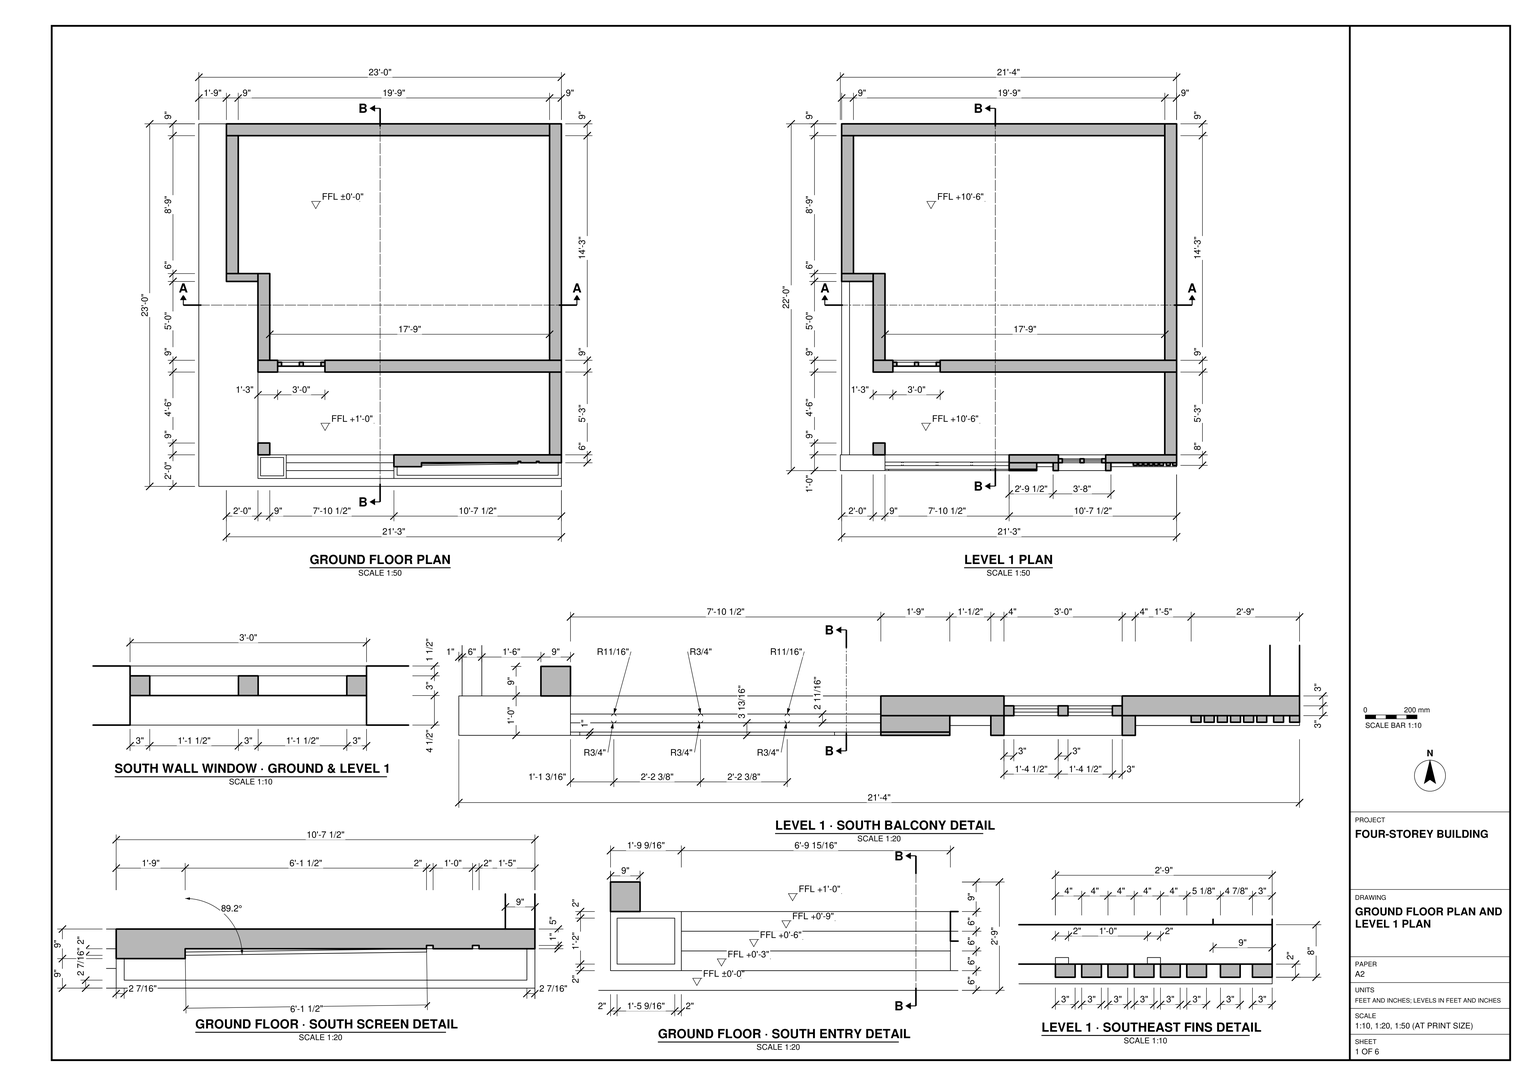
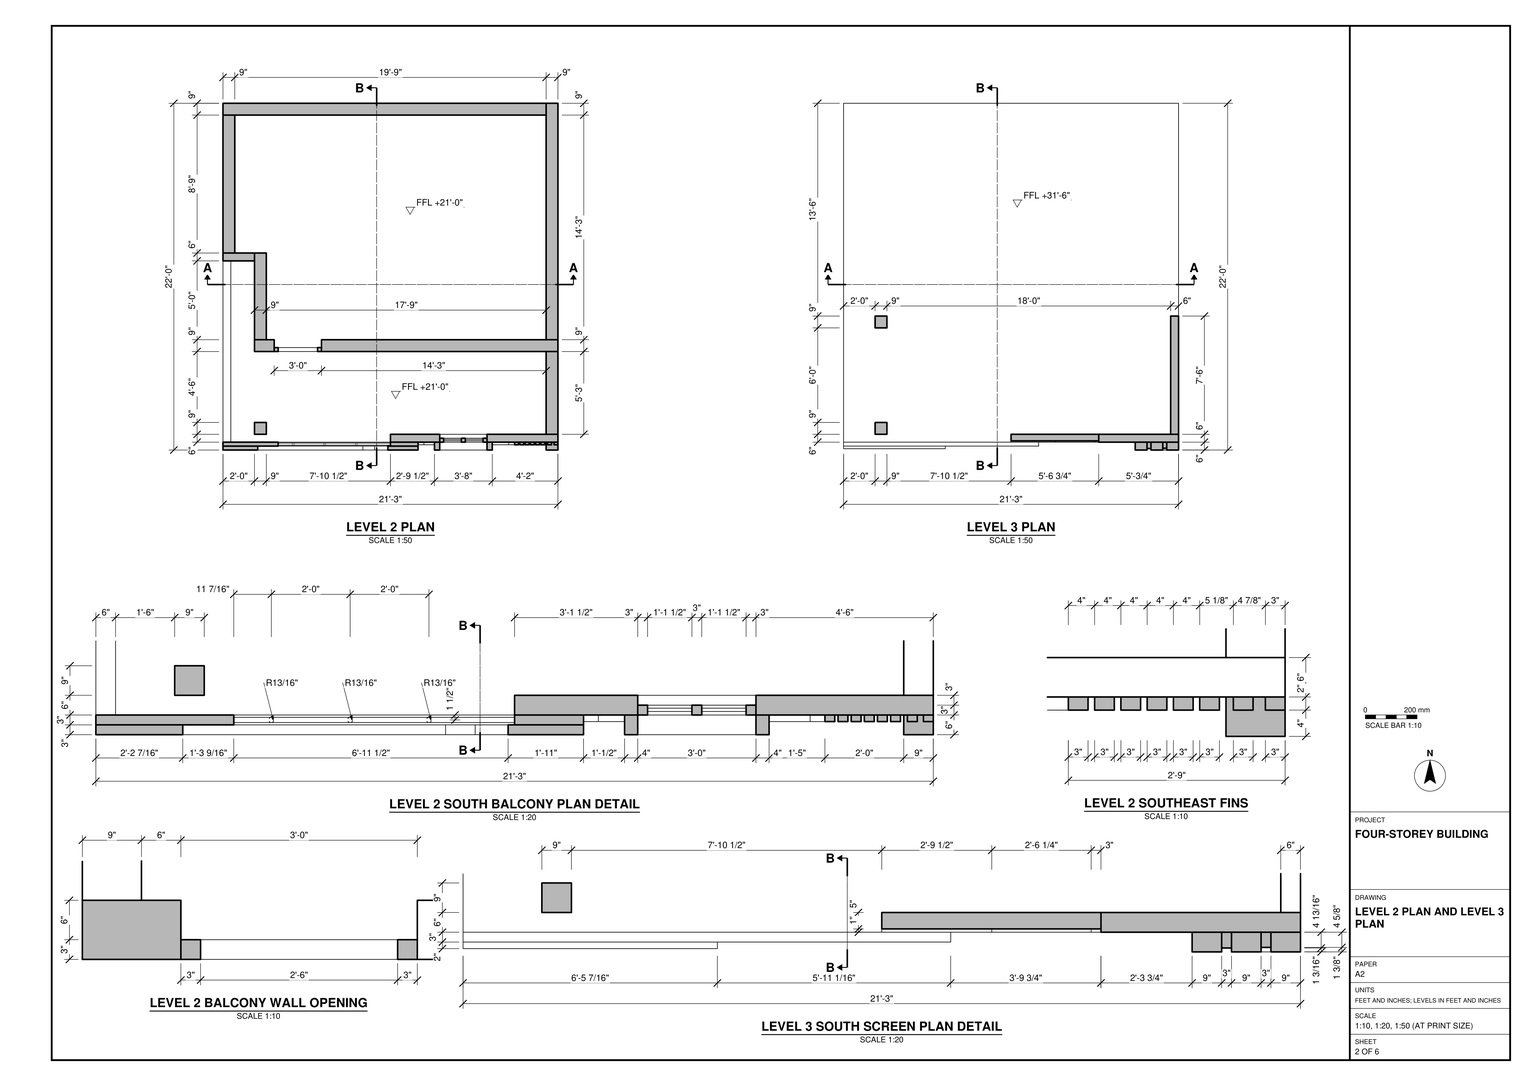
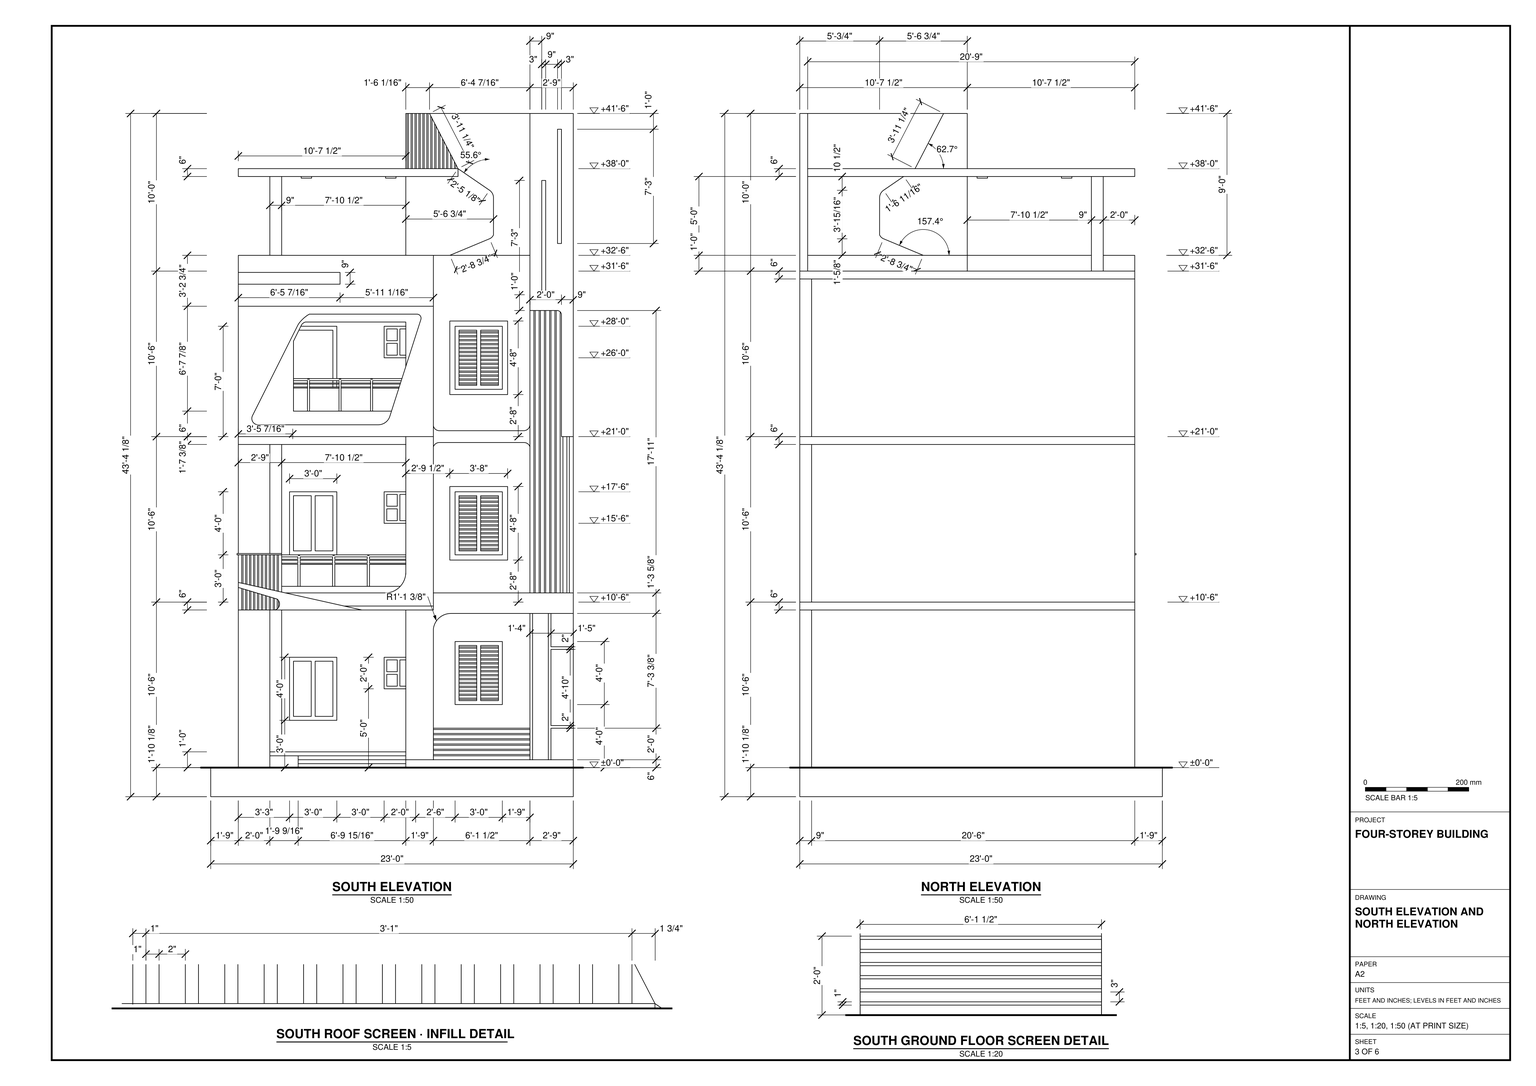
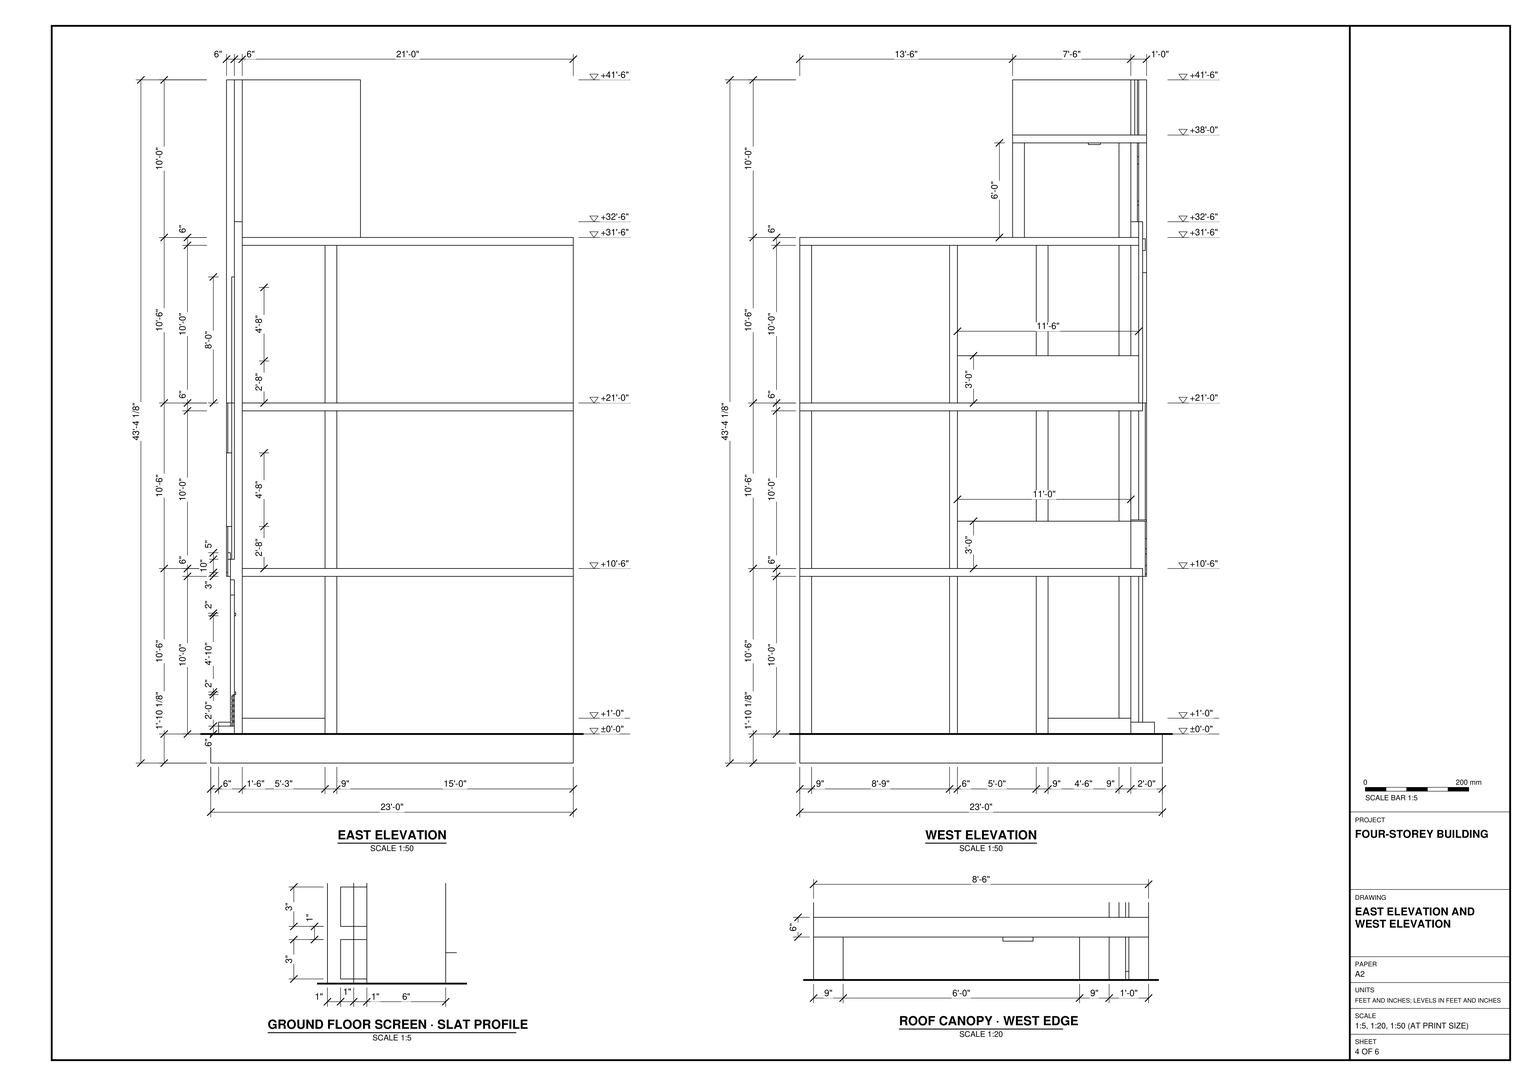
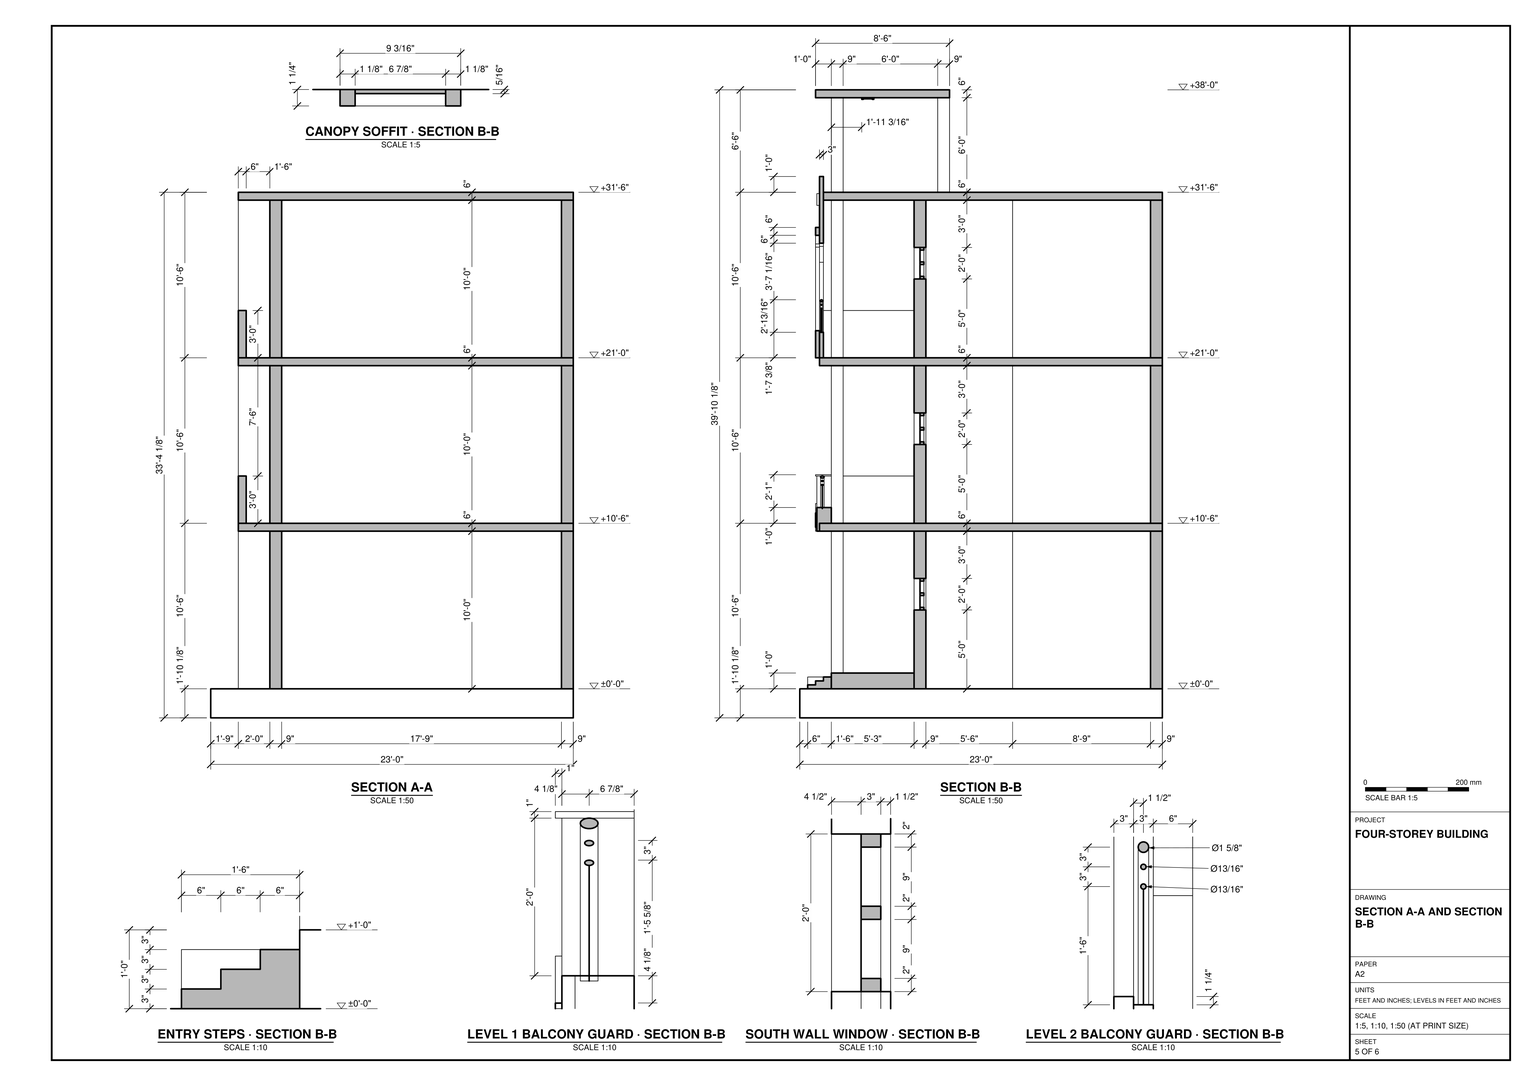
Build the four-storey building in SketchUp from task_files/diagram_01.pdf. Work in feet and inches. The overall size, from the underside of the base to the top of the roof screen, is 23'-0" wide by 23'-0" deep by 43'-4 1/8" high. Set the finished floor levels at ±0'-0", +10'-6", +21'-0" and +31'-6".

Start with the square base and use the plans to set out the slabs, walls and posts at each level. Follow the step in the west wall, using the 9" wall thickness and the 6" return where shown. On the south side, model the entry steps up to the +1'-0" landing, the recessed wall with its framed windows, and the outer screen with horizontal slats. Use the south elevation and balcony details together: the first balcony has an open railed bay, while the next has a sloping, round-cornered opening in its outer wall. Include the louvred openings and vertical fins at the east end. Keep the north wall plain below the open roof terrace, and model the terrace posts, flat canopy and raised screen.

Keep shell elements such as walls, slabs and roof, and each furniture or joinery piece shown, in separate groups or components. Use components for repeated parts. Any decor or loose items shown may be suitable library components. Save one SketchUp model as output_files/four_storey_building_with_south_balconies.skp.

# SketchUp Ruby script. Lengths in inches.
U = 1.inch
M = Sketchup.active_model
def pt(a) = Geom::Point3d.new(a.map { |v| v * U })
def face(e, loops, mat)
  f = e.add_face(loops[0].map { |a| pt(a) })
  loops[1..].each { |l| e.add_face(l.map { |a| pt(a) }).erase! }
  f.material = f.back_material = mat if mat
  f
end
# faces: each face lists its corners as indices into pts; further lists are holes
def faces(e, pts, list, mat = nil) = list.each { |f| face(e, (f[0].is_a?(Array) ? f : [f]).map { |l| l.map { |i| pts[i] } }, mat) }
# xy, xz, yz: faces in a plane at the given z, y or x. An outline is a flat list of corners, or four numbers for a rectangle; further outlines are holes
def ring(l) = l.size == 4 ? [[l[0], l[1]], [l[2], l[1]], [l[2], l[3]], [l[0], l[3]]] : l.each_slice(2).to_a
def flat(e, list, mat, &to3) = list.each { |f| face(e, (f[0].is_a?(Array) ? f : [f]).map { |l| ring(l).map { |u, v| to3.(u, v) } }, mat) }
def xy(e, z, list, mat = nil) = flat(e, list, mat) { |x, y| [x, y, z] }
def xz(e, y, list, mat = nil) = flat(e, list, mat) { |x, z| [x, y, z] }
def yz(e, x, list, mat = nil) = flat(e, list, mat) { |y, z| [x, y, z] }
def lines(e, pts, list) = list.each { |a, b| e.add_line(pt(pts[a]), pt(pts[b])) }
# prism: a flat outline (further loops are holes) pulled along v
def prism(e, loops, v, mat = nil)
  f = face(e, loops, mat); d = Geom::Vector3d.new(v.map { |x| x * U })
  f.pushpull(f.normal.samedirection?(d) ? d.length : -d.length)
end
def box(e, o, s, mat = nil) = prism(e, [[o, [o[0] + s[0], o[1], o[2]], [o[0] + s[0], o[1] + s[1], o[2]], [o[0], o[1] + s[1], o[2]]]], [0, 0, s[2]], mat)
def at(x, y, z, deg = 0) = Geom::Transformation.translation(pt([x, y, z])) * Geom::Transformation.rotation(ORIGIN, Z_AXIS, deg.degrees)
def axes(o, x, y, z) = Geom::Transformation.new([*x, 0, *y, 0, *z, 0, *pt(o).to_a, 1])
def part(name) = M.definitions.add(name)
# library, detail: a bought-in or finely detailed component or shape, given as its bounding box
def library(name, o, s) = part(name).tap { |d| box(d.entities, o, s) }
def detail(e, o, s) = box(e.add_group.entities, o, s)
def put(e, d, t, mat = nil) = e.add_instance(d, t).tap { |i| i.material = mat if mat }
def group(e, t, mat = nil) = e.add_group.tap { |g| g.transformation = t; g.material = mat if mat }.entities
root = M.entities
M.materials.add("[0047_Khaki]").color = [240, 230, 140]
M.materials.add("[0078_DarkSlateGray]").color = [47, 79, 79]
M.materials.add("[0099_LightSteelBlue]").color = [176, 196, 222]
M.materials.add("[0107_MidnightBlue]").color = [18, 18, 81]
M.materials.add("[0117_GhostWhite]").color = [248, 248, 255]
M.materials.add("[0119_RosyBrown]").color = [255, 193, 193]
M.materials.add("[0129_WhiteSmoke]").color = [245, 245, 245]
M.materials.add("[Aluminum]").color = [179, 179, 179]
M.materials.add("[Color M00]").color = [255, 255, 255]
M.materials.add("[Color M08]").color = [30, 30, 30]
M.materials.add("[Grass Dark Green]").color = [106, 157, 55]
M.materials.add("[Metal Aluminum Anodized]").color = [202, 209, 219]
M.materials.add("[Metal Rusted]").color = [184, 117, 91]
M.materials.add("[Translucent Glass Gray]").color = [0, 0, 0]
M.materials["[Translucent Glass Gray]"].alpha = 0.87
M.materials.add("[Wood Cherry Original]").color = [152, 86, 42]
M.materials.add("[Wood Veneer 02]").color = [190, 128, 91]
c1 = part("Group\#3")
box(c1.entities,[0,0,0],[24,6,120])
c2 = part("Group\#4")
box(c2.entities,[0,0,0],[9,66,120])
c3 = part("Group\#9")
prism(c3.entities,[[[231,9,0],[0,9,0],[0,9,120],[231,9,120]],[[51,9,84],[15,9,84],[15,9,36],[51,9,36]],[[111,9,84],[87,9,84],[87,9,60],[111,9,60]]],[0,-9,0])
c4 = part("Group\#6")
box(c4.entities,[0,0,0],[9,180,120])
c5 = part("Group\#7")
box(c5.entities,[0,0,0],[246,9,120])
c6 = part("Group\#2")
box(c6.entities,[0,0,0],[9,105,120])
c7 = part("Group\#17")
xz(c7.entities,0,[[3,3,16.5,45],[19.5,3,33,45]],"[Translucent Glass Gray]")
g1 = group(c7.entities,at(0,0,0),"[Wood Veneer 02]")
prism(g1,[[[0,3,0],[0,3,48],[36,3,48],[36,3,0]],[[16.5,3,3],[16.5,3,45],[3,3,45],[3,3,3]],[[33,3,45],[19.5,3,45],[19.5,3,3],[33,3,3]]],[0,-3,0])
c8 = part("Group\#11")
xz(c8.entities,0,[[2,2,10,11],[12,2,22,22],[2,13,10,22]],"[Translucent Glass Gray]")
g2 = group(c8.entities,at(0,0,0),"[Wood Veneer 02]")
prism(g2,[[[0,3,24],[24,3,24],[24,3,0],[0,3,0]],[[22,3,22],[12,3,22],[12,3,2],[22,3,2]],[[10,3,2],[10,3,11],[2,3,11],[2,3,2]],[[2,3,22],[2,3,13],[10,3,13],[10,3,22]]],[0,-3,0])
c9 = part("Group\#31")
box(c9.entities,[0,0,0],[9,9,120])
c10 = part("Group\#21")
xy(c10.entities,0,[[0,0,44,6]])
xy(c10.entities,4,[[4,0,40,6]])
xy(c10.entities,52,[[4,0,40,6]])
xy(c10.entities,56,[[0,0,44,6]])
xz(c10.entities,0,[[[0,0,44,56],[4,4,40,52]]],"[Wood Cherry Original]")
xz(c10.entities,6,[[[0,0,44,56],[4,4,40,52]]])
yz(c10.entities,0,[[0,0,6,56]])
yz(c10.entities,4,[[0,4,6,52]])
yz(c10.entities,40,[[0,4,6,52]])
yz(c10.entities,44,[[0,0,6,56]])
c11 = part("Group\#23")
prism(c11.entities,[[[0,0.98,0.37],[0,0.93,0.25],[0,0.85,0.15],[0,0.75,0.07],[0,0.63,0.02],[0,0.5,0],[0,0.37,0.02],[0,0.25,0.07],[0,0.15,0.15],[0,0.07,0.25],[0,0.02,0.37],[0,0,0.5],[0,0.02,0.63],[0,0.07,0.75],[0,0.15,0.85],[0,0.25,0.93],[0,0.37,0.98],[0,0.5,1],[0,0.63,0.98],[0,0.75,0.93],[0,0.85,0.85],[0,0.93,0.75],[0,0.98,0.63],[0,1,0.5]]],[33.3125,0,0])
c12 = part("Group\#20")
g3 = group(c12.entities,at(0,0,0),"[Color M08]")
prism(g3,[[[0,3,0],[0,3,48],[36,3,48],[36,3,0]],[[16.5,3,3],[16.5,3,45],[3,3,45],[3,3,3]],[[33,3,45],[19.5,3,45],[19.5,3,3],[33,3,3]]],[0,-3,0])
put(c12.entities,c11,at(2,1.07,6.91),"[Aluminum]")
put(c12.entities,c11,at(2,1.07,15.91),"[Aluminum]")
put(c12.entities,c11,at(2,1.07,30.91),"[Aluminum]")
put(c12.entities,c11,at(2,1.07,3.91),"[Aluminum]")
put(c12.entities,c11,at(2,1.07,39.91),"[Aluminum]")
put(c12.entities,c11,at(2,1.07,36.91),"[Aluminum]")
put(c12.entities,c11,at(2,1.07,42.91),"[Aluminum]")
put(c12.entities,c11,at(2,1.07,9.91),"[Aluminum]")
put(c12.entities,c11,at(2,1.07,24.91),"[Aluminum]")
put(c12.entities,c11,at(2,1.07,27.91),"[Aluminum]")
put(c12.entities,c11,at(2,1.07,12.91),"[Aluminum]")
put(c12.entities,c11,at(2,1.07,33.91),"[Aluminum]")
put(c12.entities,c11,at(2,1.07,18.91),"[Aluminum]")
put(c12.entities,c11,at(2,1.07,21.91),"[Aluminum]")
c13 = part("Group\#35")
box(c13.entities,[0,0,0],[1,2,42])
c14 = library("Group\#39",[192.125,0,0],[88.3125,1.6,24.79])
c15 = part("Group\#47")
box(c15.entities,[0,0,0],[3,2,215])
c16 = part("Group\#55")
xy(c16.entities,0,[[[0,0,7.9375,9.1875],[1.15,1.15,6.79,8.04]]],"[Metal Rusted]")
xy(c16.entities,0.9375,[[1.15,1.15,6.79,8.04]],"[Metal Aluminum Anodized]")
xy(c16.entities,1.25,[[[0,0,7.9375,9.1875],[1.15,1.15,6.79,8.04]]])
xz(c16.entities,0,[[0,0,7.9375,1.25]],"[Metal Rusted]")
xz(c16.entities,1.15,[[1.15,0.9375,6.79,1.25]])
xz(c16.entities,1.15,[[1.15,0,6.79,0.9375]],"[Metal Rusted]")
xz(c16.entities,8.04,[[1.15,0.9375,6.79,1.25]])
xz(c16.entities,8.04,[[1.15,0,6.79,0.9375]],"[Metal Rusted]")
xz(c16.entities,9.1875,[[0,0,7.9375,1.25]],"[Metal Rusted]")
yz(c16.entities,0,[[0,0,9.1875,1.25]])
yz(c16.entities,1.15,[[1.15,0.9375,8.04,1.25]])
yz(c16.entities,1.15,[[1.15,0,8.04,0.9375]],"[Metal Rusted]")
yz(c16.entities,6.79,[[1.15,0.9375,8.04,1.25]])
yz(c16.entities,6.79,[[1.15,0,8.04,0.9375]],"[Metal Rusted]")
yz(c16.entities,7.9375,[[0,0,9.1875,1.25]],"[Metal Rusted]")
xy(root,24.125,[[150.9375,8.4375,273.5625,8.4375,273.5625,18,148.5,18,148.5,15,150.9375,15]],"[Grass Dark Green]")
xy(root,28.125,[[148.5,6,276,6,276,18,273.5625,18,273.5625,8.4375,150.9375,8.4375,150.9375,15,148.5,15]])
xz(root,6,[[148.5,22.125,276,28.125]])
xz(root,8.4375,[[150.9375,24.125,273.5625,28.125]])
xz(root,15,[[148.5,24.125,150.9375,28.125]])
xz(root,18,[[148.5,22.125,273.5625,24.125],[273.5625,22.125,276,28.125]])
yz(root,148.5,[[6,22.125,15,28.125],[15,22.125,18,24.125]])
yz(root,150.9375,[[8.4375,24.125,15,28.125]])
yz(root,273.5625,[[8.4375,24.125,15.5625,28.125],[15.5625,24.125,18,28.125]])
yz(root,276,[[6,22.125,18,28.125]])
# 3 loose lines left out
g4 = group(root,at(36,96,0))
box(g4,[-36,-96,0],[276,276,22.125])
put(root,c1,at(21,156,22.125),"[0117_GhostWhite]")
put(root,c2,at(45,96,22.125),"[0117_GhostWhite]")
put(root,c3,at(45,87,22.125),"[0117_GhostWhite]")
put(root,c4,at(267,96,22.125),"[0117_GhostWhite]")
put(root,c5,at(21,267,22.125),"[0117_GhostWhite]")
put(root,c6,at(21,162,22.125),"[0117_GhostWhite]")
put(root,c7,at(60,91.5,58.125))
put(root,c8,at(132,91.5,82.125))
g5 = group(root,at(21,24,142.125),"[0117_GhostWhite]")
prism(g5,[[[0,-9,0],[0,252,0],[255,252,0],[255,0,0],[127.5,0,0],[127.5,-9,0]]],[0,0,6])
put(root,c6,at(21,162,148.125),"[0117_GhostWhite]")
put(root,c2,at(45,96,148.125),"[0117_GhostWhite]")
put(root,c8,at(132,91.5,208.125))
put(root,c9,at(45,24,148.125),"[0117_GhostWhite]")
put(root,c1,at(21,156,148.125),"[0117_GhostWhite]")
put(root,c5,at(21,267,148.125),"[0117_GhostWhite]")
g6 = group(root,at(21,24,268.125),"[0117_GhostWhite]")
prism(g6,[[[0,-9,0],[0,252,0],[255,252,0],[255,0,0],[127.5,0,0],[127.5,-9,0]]],[0,0,6])
put(root,c7,at(60,91.5,184.125))
put(root,c4,at(267,96,148.125),"[0117_GhostWhite]")
g7 = group(root,at(45,6,22.125),"[0117_GhostWhite]")
xy(g7,0,[[21.5625,0,103.5,18],[0,18,231,81]])
xy(g7,3,[[21.5625,0,103.5,6]])
xy(g7,6,[[21.5625,6,103.5,12]])
xy(g7,9,[[21.5625,12,103.5,18]])
xy(g7,12,[[0,18,231,81]])
xz(g7,0,[[21.5625,0,103.5,3]])
xz(g7,6,[[21.5625,3,103.5,6]])
xz(g7,12,[[21.5625,6,103.5,9]])
xz(g7,18,[[0,0,21.5625,0,21.5625,9,231,9,231,12,0,12],[21.5625,0,103.5,9],[103.5,0,231,9]])
xz(g7,81,[[0,0,231,12]])
yz(g7,0,[[18,0,81,12]])
yz(g7,21.5625,[[0,0,0,3,6,3,6,6,12,6,12,9,18,9,18,0]])
yz(g7,103.5,[[0,0,18,0,18,9,12,9,12,6,6,6,6,3,0,3]])
yz(g7,231,[[18,0,81,12]])
g8 = group(root,at(45,24,34.125),"[0117_GhostWhite]")
box(g8,[0,0,0],[9,9,108])
put(root,c6,at(21,162,274.125),"[0117_GhostWhite]")
put(root,c1,at(21,156,274.125),"[0117_GhostWhite]")
put(root,c5,at(21,267,274.125),"[0117_GhostWhite]")
g9 = group(root,at(21,24,394.125),"[0117_GhostWhite]")
prism(g9,[[[0,-6,0],[0,252,0],[255,252,0],[255,0,0],[127.5,0,0],[127.5,-6,0]]],[0,0,6])
put(root,c4,at(267,96,274.125),"[0117_GhostWhite]")
put(root,c2,at(45,96,274.125),"[0117_GhostWhite]")
g10 = group(root,at(45,87,274.125),"[0117_GhostWhite]")
g11 = group(g10,at(15,0,0),"[Wood Veneer 02]")
prism(g11,[[[0,0,0],[36,0,0],[36,0,84],[0,0,84]],[[33,0,81],[33,0,3],[3,0,3],[3,0,81]]],[0,3,0])
g12 = group(g10,at(0,0,0))
g13 = group(g12,at(0,0,0))
prism(g13,[[[51,0,84],[51,0,0],[231,0,0],[231,0,120],[0,0,120],[0,0,0],[15,0,0],[15,0,84]],[[87,0,84],[111,0,84],[111,0,60],[87,0,60]]],[0,9,0])
put(g12,c8,at(87,4.5,60))
put(root,c10,at(182,12,180.125))
put(root,c3,at(45,87,148.125),"[0117_GhostWhite]")
put(root,c12,at(186,18,184.125))
put(root,c12,at(186,18,70.125))
put(root,c12,at(186,18,310.125))
put(root,c10,at(182,12,306.125))
g14 = group(root,at(45,24,400.125),"[0117_GhostWhite]")
box(g14,[0,0,0],[9,9,72])
g15 = group(root,at(45,105,400.125),"[0117_GhostWhite]")
box(g15,[0,0,0],[9,9,72])
g16 = group(root,at(270,24,400.125),"[0117_GhostWhite]")
box(g16,[0,0,0],[6,90,120])
g17 = group(root,at(21,15,274.125),"[0119_RosyBrown]")
xy(g17,-119,[[127.5,-2,148.5,3]])
xy(g17,0,[[127.5,-2,148.5,0],[0,0,127.5,3]])
xy(g17,19.38,[[42,0,127.5,3]])
xy(g17,87.23,[[51,0,127.5,3]])
xy(g17,138,[[0,0,148.5,3]])
xz(g17,-2,[[127.5,-119,148.5,0]])
xz(g17,0,[[[0,0,148.5,138],[42,19.38,42,72.69,48,84.81,48.15,85.08,48.31,85.34,48.5,85.59,48.71,85.83,48.94,86.05,49.19,86.27,49.46,86.47,49.74,86.65,50.04,86.82,50.35,86.98,50.67,87.11,51,87.23,127.5,87.23,127.5,19.38]]])
xz(g17,3,[[[127.5,-119,127.5,0,0,0,0,138,148.5,138,148.5,-119],[42,19.38,127.5,19.38,127.5,87.23,51,87.23,50.67,87.11,50.35,86.98,50.04,86.82,49.74,86.65,49.46,86.47,49.19,86.27,48.94,86.05,48.71,85.83,48.5,85.59,48.31,85.34,48.15,85.08,48,84.81,42,72.69]]])
yz(g17,0,[[0,0,3,138]])
yz(g17,42,[[0,19.38,3,72.69]])
yz(g17,127.5,[[-2,-119,3,0],[0,19.38,3,87.23]])
yz(g17,148.5,[[-2,-119,3,-119,3,138,0,138,0,0,-2,0]])
p = [[42,3,72.69],[48,3,84.81],[48,0,84.81],[42,0,72.69],[48.15,3,85.08],[48.15,0,85.08],
  [48.31,3,85.34],[48.31,0,85.34],[48.5,3,85.59],[48.5,0,85.59],[48.71,3,85.83],[48.71,0,85.83],
  [48.94,3,86.05],[48.94,0,86.05],[49.19,3,86.27],[49.19,0,86.27],[49.46,3,86.47],[49.46,0,86.47],
  [49.74,3,86.65],[49.74,0,86.65],[50.04,3,86.82],[50.04,0,86.82],[50.35,3,86.98],[50.35,0,86.98],
  [50.67,3,87.11],[50.67,0,87.11],[51,3,87.23],[51,0,87.23]]
faces(g17,p,[[0,1,2,3],[1,4,5,2],[4,6,7,5],[6,8,9,7],[8,10,11,9],[10,12,13,11],[12,14,15,13],[14,16,17,15],
  [16,18,19,17],[18,20,21,19],[20,22,23,21],[22,24,25,23],[24,26,27,25]])
g18 = group(root,at(21,12,274.125),"[Wood Cherry Original]")
prism(g18,[[[148.5,3,99.23],[148.5,3,0],[0,3,0],[0,3,99.23]],[[47.04,3,87.33],[46.51,3,86.68],[46.08,3,86.1],[45.68,3,85.5],[45.32,3,84.875],[45,3,84.23],[10.78,3,15.95],[10.48,3,15.21],[10.31,3,14.43],[10.27,3,13.63],[10.37,3,12.84],[10.59,3,12.07],[10.9375,3,11.35],[11.4,3,10.7],[11.97,3,10.14],[12.62,3,9.67],[13.34,3,9.32],[14.1,3,9.1],[14.9,3,9],[106.5,3,9],[107.52,3,9.06],[108.52,3,9.22],[109.5,3,9.5],[110.45,3,9.88],[111.35,3,10.36],[112.1875,3,10.94],[112.96,3,11.61],[113.65,3,12.35],[114.26,3,13.17],[114.77,3,14.05],[115.1875,3,14.98],[115.5,3,15.95],[136.24,3,80.65],[137.38,3,84.23],[138.97,3,89.17],[139.08,3,89.625],[139.12,3,90.09],[139.08,3,90.56],[138.98,3,91.02],[138.82,3,91.46],[138.58,3,91.86],[138.29,3,92.23],[137.95,3,92.55],[137.57,3,92.82],[137.15,3,93.02],[136.7,3,93.16],[136.24,3,93.23],[54,3,93.23],[53.29,3,92.79],[52.59,3,92.34],[51.91,3,91.86],[51.24,3,91.36],[50.59,3,90.84],[49.95,3,90.3],[49.33,3,89.74],[48.73,3,89.17],[48.15,3,88.57],[47.58,3,87.96]]],[0,-3,0])
g19 = group(root,at(21,12,472.125))
xy(g19,0,[[0,0,0,102,249,102,249,12,167.25,12,167.25,0]])
xy(g19,6,[[0,0,167.25,0,167.25,12,249,12,249,102,0,102]])
xz(g19,0,[[0,0,167.25,6]],"[Wood Cherry Original]")
xz(g19,12,[[167.25,0,249,6]])
xz(g19,102,[[0,0,249,6]])
yz(g19,0,[[0,0,102,6]])
yz(g19,167.25,[[0,0,12,6]])
yz(g19,249,[[12,0,71.3125,6],[71.3125,0,102,6]])
g20 = group(root,at(21,13,390.13),"[0107_MidnightBlue]")
box(g20,[0,0,0],[77.4375,2,9])
g21 = group(root,at(148.5,24,412.125),"[0047_Khaki]")
xy(g21,0,[[33.5,-6,127.5,0],[0,-5,33.5,0]],"[0119_RosyBrown]")
xy(g21,60,[[0,-5,39.75,-3]],"[0119_RosyBrown]")
xy(g21,108,[[18.05,-6,127.5,0],[0,-3,18.05,0]],"[0119_RosyBrown]")
xz(g21,-6,[[33.5,0,63.75,12.62,64.08,12.77,64.4,12.9375,64.71,13.13,65,13.34,65.28,13.57,65.55,13.82,65.79,14.09,66.02,14.37,66.24,14.66,66.43,14.97,66.6,15.29,66.75,15.62,66.75,43.8,66.73,44.37,66.67,44.92,66.56,45.47,66.4,46.01,66.2,46.54,65.96,47.05,65.68,47.53,65.36,47.99,65.01,48.43,64.62,48.83,64.2,49.2,63.75,49.54,39.75,66,18.05,108,127.5,108,127.5,0]],"[0119_RosyBrown]")
xz(g21,-3,[[0,60,39.75,60,39.75,66,18.05,108,0,108]],"[0119_RosyBrown]")
xz(g21,0,[[0,0,0,108,18.05,108,39.75,66,63.75,49.54,64.2,49.2,64.62,48.83,65.01,48.43,65.36,47.99,65.68,47.53,65.96,47.05,66.2,46.54,66.4,46.01,66.56,45.47,66.67,44.92,66.73,44.37,66.75,43.8,66.75,15.62,66.6,15.29,66.43,14.97,66.24,14.66,66.02,14.37,65.79,14.09,65.55,13.82,65.28,13.57,65,13.34,64.71,13.13,64.4,12.9375,64.08,12.77,63.75,12.62,33.5,0],[33.5,0,63.75,12.62,64.08,12.77,64.4,12.9375,64.71,13.13,65,13.34,65.28,13.57,65.55,13.82,65.79,14.09,66.02,14.37,66.24,14.66,66.43,14.97,66.6,15.29,66.75,15.62,66.75,43.8,66.73,44.37,66.67,44.92,66.56,45.47,66.4,46.01,66.2,46.54,65.96,47.05,65.68,47.53,65.36,47.99,65.01,48.43,64.62,48.83,64.2,49.2,63.75,49.54,39.75,66,18.05,108,127.5,108,127.5,0]],"[0119_RosyBrown]")
yz(g21,0,[[-5,0,-5,60,-3,60,-3,108,0,108,0,0]],"[0119_RosyBrown]")
yz(g21,39.75,[[-5,60,-3,60.0625],[-5,60.0625,-3,66]],"[0119_RosyBrown]")
yz(g21,66.75,[[-6,15.62,-5,43.8],[-5,15.62,0,43.8]],"[0119_RosyBrown]")
yz(g21,127.5,[[-6,0,0,108]],"[0119_RosyBrown]")
p = [[33.5,-6,0],[63.75,-6,12.62],[63.75,-5,12.62],[33.5,-5,0],[63.75,0,12.62],[33.5,0,0],
  [64.08,-6,12.77],[64.08,-5,12.77],[64.08,0,12.77],[64.4,-6,12.9375],[64.4,-5,12.9375],[64.4,0,12.9375],
  [64.71,-6,13.13],[64.71,-5,13.13],[64.71,0,13.13],[65,-6,13.34],[65,-5,13.34],[65,0,13.34],
  [65.28,-6,13.57],[65.28,-5,13.57],[65.28,0,13.57],[65.55,-6,13.82],[65.55,-5,13.82],[65.55,0,13.82],
  [65.79,-6,14.09],[65.79,-5,14.09],[65.79,0,14.09],[66.02,-6,14.37],[66.02,-5,14.37],[66.02,0,14.37],
  [66.24,-6,14.66],[66.24,-5,14.66],[66.24,0,14.66],[66.43,-6,14.97],[66.43,-5,14.97],[66.43,0,14.97],
  [66.6,-6,15.29],[66.6,-5,15.29],[66.6,0,15.29],[66.75,-6,15.62],[66.75,-5,15.62],[66.75,0,15.62],
  [66.73,-6,44.37],[66.73,-5,44.37],[66.75,-5,43.8],[66.75,-6,43.8],[66.73,0,44.37],[66.75,0,43.8],
  [66.67,-6,44.92],[66.67,-5,44.92],[66.67,0,44.92],[66.56,-6,45.47],[66.56,-5,45.47],[66.56,0,45.47],
  [66.4,-6,46.01],[66.4,-5,46.01],[66.4,0,46.01],[66.2,-6,46.54],[66.2,-5,46.54],[66.2,0,46.54],
  [65.96,-6,47.05],[65.96,-5,47.05],[65.96,0,47.05],[65.68,-6,47.53],[65.68,-5,47.53],[65.68,0,47.53],
  [65.36,-6,47.99],[65.36,-5,47.99],[65.36,0,47.99],[65.01,-6,48.43],[65.01,-5,48.43],[65.01,0,48.43],
  [64.62,-6,48.83],[64.62,-5,48.83],[64.62,0,48.83],[64.2,-6,49.2],[64.2,-5,49.2],[64.2,0,49.2],
  [63.75,-6,49.54],[63.75,-5,49.54],[63.75,0,49.54],[39.75,-6,66],[39.75,-5,66],[39.75,0,66],
  [39.75,-3,66],[18.05,-6,108],[18.05,-3,108],[18.05,0,108]]
faces(g21,p,[[0,1,2,3],[4,5,3,2],[1,6,7,2],[8,4,2,7],[6,9,10,7],[11,8,7,10],[9,12,13,10],[14,11,10,13],
  [15,16,13,12],[17,14,13,16],[18,19,16,15],[20,17,16,19],[21,22,19,18],[23,20,19,22],[24,25,22,21],[26,23,22,25],
  [27,28,25,24],[29,26,25,28],[30,31,28,27],[32,29,28,31],[33,34,31,30],[35,32,31,34],[36,37,34,33],[38,35,34,37],
  [39,40,37,36],[41,38,37,40],[42,43,44,45],[46,47,44,43],[48,49,43,42],[50,46,43,49],[51,52,49,48],[53,50,49,52],
  [54,55,52,51],[56,53,52,55],[57,58,55,54],[59,56,55,58],[60,61,58,57],[62,59,58,61],[63,64,61,60],[65,62,61,64],
  [66,67,64,63],[68,65,64,67],[69,70,67,66],[71,68,67,70],[72,73,70,69],[74,71,70,73],[75,76,73,72],[77,74,73,76],
  [78,79,76,75],[80,77,76,79],[81,82,79,78],[83,80,79,82,84],[85,86,84,82,81],[87,83,84,86]],"[0119_RosyBrown]")
g22 = group(g21,at(0,-5,0))
xz(g22,0,[[0,0,33.5,0,63.75,12.62,64.08,12.77,64.4,12.9375,64.71,13.13,65,13.34,65.28,13.57,65.55,13.82,65.79,14.09,66.02,14.37,66.24,14.66,66.43,14.97,66.6,15.29,66.75,15.62,66.75,43.8,66.73,44.37,66.67,44.92,66.56,45.47,66.4,46.01,66.2,46.54,65.96,47.05,65.68,47.53,65.36,47.99,65.01,48.43,64.62,48.83,64.2,49.2,63.75,49.54,39.75,66,39.75,60,0,60]],"[Color M00]")
g23 = group(root,at(149.5,19,478.125),"[0119_RosyBrown]")
put(g23,c13,at(6,0,0))
put(g23,c13,at(12,0,0))
put(g23,c13,at(0,0,0))
put(g23,c13,at(30,0,0))
put(g23,c13,at(9,0,0))
put(g23,c13,at(33,0,0))
put(g23,c13,at(3,0,0))
put(g23,c13,at(27,0,0))
put(g23,c13,at(15,0,0))
put(g23,c13,at(18,0,0))
put(g23,c13,at(21,0,0))
put(g23,c13,at(36,0,0))
put(g23,c13,at(24,0,0))
put(root,c14,at(-129.6875,15.7,293.51))
g24 = group(root,at(21,18,274.125),"[0117_GhostWhite]")
box(g24,[0,0,0],[6,138,36])
g25 = group(root,at(21,24,148.125),"[0117_GhostWhite]")
box(g25,[0,0,0],[6,132,36])
put(root,c9,at(45,24,274.125))
g26 = group(root,at(21,15,148.125),"[0119_RosyBrown]")
xy(g26,-6,[[0,-2,0,0,33,0,33,-2,30.56,-2,30.56,-1,29.56,-1,29.56,-2,27.56,-2,27.56,-1,26.56,-1,26.56,-2,24.56,-2,24.56,-1,23.56,-1,23.56,-2,21.56,-2,21.56,-1,20.56,-1,20.56,-2,18.56,-2,18.56,-1,17.56,-1,17.56,-2,15.56,-2,15.56,-1,14.56,-1,14.56,-2,12.56,-2,12.56,-1,11.56,-1,11.56,-2,9.56,-2,9.56,-1,8.56,-1,8.56,-2,6.56,-2,6.56,-1,5.56,-1,5.56,-2,3.56,-2,3.56,-1,2.56,-1,2.56,-2],[33,-2,148.5,0]],"[0047_Khaki]")
xy(g26,0,[[0,0,127.5,9]],"[0047_Khaki]")
xy(g26,12,[[33,-2,148.5,-2,148.5,0,127.5,0,127.5,9,33,9]])
xy(g26,36,[[0,-2,2.56,-2,2.56,-1,3.56,-1,3.56,-2,5.56,-2,5.56,-1,6.56,-1,6.56,-2,8.56,-2,8.56,-1,9.56,-1,9.56,-2,11.56,-2,11.56,-1,12.56,-1,12.56,-2,14.56,-2,14.56,-1,15.56,-1,15.56,-2,17.56,-2,17.56,-1,18.56,-1,18.56,-2,20.56,-2,20.56,-1,21.56,-1,21.56,-2,23.56,-2,23.56,-1,24.56,-1,24.56,-2,26.56,-2,26.56,-1,27.56,-1,27.56,-2,29.56,-2,29.56,-1,30.56,-1,30.56,-2,33,-2,33,9,0,9]],"[0047_Khaki]")
xz(g26,-2,[[33,-6,148.5,12]])
xz(g26,-2,[[0,-6,2.56,36],[3.56,-6,5.56,36],[6.56,-6,8.56,36],[9.56,-6,11.56,36],[12.56,-6,14.56,36],
  [15.56,-6,17.56,36],[18.56,-6,20.56,36],[21.56,-6,23.56,36],[24.56,-6,26.56,36],[27.56,-6,29.56,36],
  [30.56,-6,33,36]],"[0047_Khaki]")
xz(g26,-1,[[2.56,-6,3.56,36],[5.56,-6,6.56,36],[8.56,-6,9.56,36],[11.56,-6,12.56,36],[14.56,-6,15.56,36],
  [17.56,-6,18.56,36],[20.56,-6,21.56,36],[23.56,-6,24.56,36],[26.56,-6,27.56,36],[29.56,-6,30.56,36]],"[0047_Khaki]")
xz(g26,0,[[0,-6,33,0],[33,-6,148.5,0],[127.5,0,148.5,12]],"[0047_Khaki]")
xz(g26,9,[[0,0,0,36,33,36,33,12,127.5,12,127.5,0]],"[0047_Khaki]")
yz(g26,0,[[-2,-6,-2,36,9,36,9,0,0,0,0,-6]],"[0047_Khaki]")
yz(g26,2.56,[[-2,-6,-1,36]],"[0047_Khaki]")
yz(g26,3.56,[[-2,-6,-1,36]],"[0047_Khaki]")
yz(g26,5.56,[[-2,-6,-1,36]],"[0047_Khaki]")
yz(g26,6.56,[[-2,-6,-1,36]],"[0047_Khaki]")
yz(g26,8.56,[[-2,-6,-1,36]],"[0047_Khaki]")
yz(g26,9.56,[[-2,-6,-1,36]],"[0047_Khaki]")
yz(g26,11.56,[[-2,-6,-1,36]],"[0047_Khaki]")
yz(g26,12.56,[[-2,-6,-1,36]],"[0047_Khaki]")
yz(g26,14.56,[[-2,-6,-1,36]],"[0047_Khaki]")
yz(g26,15.56,[[-2,-6,-1,36]],"[0047_Khaki]")
yz(g26,17.56,[[-2,-6,-1,36]],"[0047_Khaki]")
yz(g26,18.56,[[-2,-6,-1,36]],"[0047_Khaki]")
yz(g26,20.56,[[-2,-6,-1,36]],"[0047_Khaki]")
yz(g26,21.56,[[-2,-6,-1,36]],"[0047_Khaki]")
yz(g26,23.56,[[-2,-6,-1,36]],"[0047_Khaki]")
yz(g26,24.56,[[-2,-6,-1,36]],"[0047_Khaki]")
yz(g26,26.56,[[-2,-6,-1,36]],"[0047_Khaki]")
yz(g26,27.56,[[-2,-6,-1,36]],"[0047_Khaki]")
yz(g26,29.56,[[-2,-6,-1,36]],"[0047_Khaki]")
yz(g26,30.56,[[-2,-6,-1,36]],"[0047_Khaki]")
yz(g26,33,[[-2,12,9,36]])
yz(g26,33,[[-2,-6,0,12]],"[0047_Khaki]")
yz(g26,127.5,[[0,0,9,12]],"[0047_Khaki]")
yz(g26,148.5,[[-2,-6,0,12]])
g27 = group(root,at(21,12,142.125),"[0099_LightSteelBlue]")
prism(g27,[[[29.56,0,0],[33,0,0],[94.07,0,0],[0,0,21],[0,0,17.17],[29.56,0,8.31],[30.01,0,7.91],[30.4,0,7.46],[30.74,0,6.96],[31.01,0,6.42],[31.21,0,5.86],[31.34,0,5.27],[31.39,0,4.68],[31.37,0,4.08],[31.27,0,3.49],[31.11,0,2.91],[30.87,0,2.36],[30.56,0,1.85],[30.38,0,1.6],[30.18,0,1.37],[29.97,0,1.16],[29.75,0,0.96],[29.51,0,0.77],[29.26,0,0.6],[28.99,0,0.45],[28.72,0,0.32],[28.44,0,0.21],[28.15,0,0.12],[27.86,0,0.05],[27.56,0,0]]],[0,1,0])
g28 = group(root,at(56.84,12,145.125),"[0078_DarkSlateGray]")
prism(g28,[[[0,1,10],[77.57,1,10],[79.47,1,10.33],[81.3125,1,10.89],[83.08,1,11.66],[84.73,1,12.65],[86.26,1,13.83],[87.625,1,15.18],[88.82,1,16.69],[89.82,1,18.34],[90.62,1,20.09],[91.2,1,21.93],[91.55,1,23.83],[91.66,1,25.75],[91.66,1,129],[112.66,1,129],[112.66,1,0],[44.8,1,0]]],[0,-1,0],"[0107_MidnightBlue]")
g29 = group(root,at(243,16,155.125),"[0107_MidnightBlue]")
put(g29,c15,at(4,0,0))
put(g29,c15,at(12,0,0))
put(g29,c15,at(8,0,0))
put(g29,c15,at(16,0,0))
put(g29,c15,at(20,0,0))
put(g29,c15,at(0,0,0))
put(g29,c15,at(25.125,0,0))
put(g29,c15,at(30,0,0))
g30 = group(root,at(148.5,18,22.125),"[0099_LightSteelBlue]")
xy(g30,0,[[0,-3,0,6,127.5,6,127.5,0,110.5,0,110.5,1,108.5,1,108.5,0,96.5,0,96.5,1,94.5,1,94.5,0,21,0,21,-3]])
xy(g30,30,[[110.5,0,127.5,1]])
xy(g30,32,[[110.5,0,127.5,1]])
xy(g30,48,[[37.5,0,73.5,6]])
xy(g30,90,[[110.5,0,127.5,1]])
xy(g30,92,[[110.5,0,127.5,1]])
xy(g30,96,[[37.5,0,73.5,6]])
xy(g30,117.37,[[34.25,-3,34.25,0,94.5,0,94.5,1,96.5,1,96.5,0,108.5,0,108.5,1,110.5,1,110.5,0,127.5,0,127.5,-3]])
xy(g30,133,[[0,-3,127.5,0]],"[Wood Cherry Original]")
xy(g30,162,[[37.5,0,73.5,6]])
xy(g30,210,[[37.5,0,73.5,6]])
xy(g30,247.5,[[25.5,-2,54.125,0],[54.125,-2,90,0]])
xy(g30,256.5,[[25.5,-2,50.85,0],[50.85,-2,90,0]])
xy(g30,288,[[37.5,0,73.5,6]])
xy(g30,336,[[37.5,0,73.5,6]])
xy(g30,390,[[0,0,127.5,6]])
xz(g30,-3,[[0,0,21,0,21,105.8,21.31,107.37,21.8,108.89,22.48,110.34,23.32,111.7,24.32,112.95,25.45,114.07,26.72,115.05,28.09,115.87,29.55,116.52,31.08,116.99,32.65,117.27,34.25,117.37,127.5,117.37,127.5,133,0,133]],"[Wood Cherry Original]")
xz(g30,-2,[[21,244.2,21.17,244.67,21.4,245.11,21.66,245.53,21.98,245.92,22.33,246.27,22.71,246.59,23.125,246.86,23.57,247.09,24.03,247.27,24.51,247.4,25,247.47,25.5,247.5,90,247.5,90.5,247.47,90.99,247.4,91.47,247.27,91.93,247.09,92.37,246.86,92.79,246.59,93.17,246.28,93.52,245.93,93.83,245.54,94.1,245.12,94.32,244.68,94.5,244.21,94.5,261.24,94.46,260.64,94.35,260.05,94.16,259.48,93.9,258.94,93.58,258.43,93.2,257.97,92.76,257.57,92.27,257.22,91.74,256.93,91.18,256.71,90.6,256.57,90,256.5,25.5,256.5,24.97,256.53,24.45,256.62,23.94,256.77,23.46,256.98,23,257.24,22.57,257.56,22.1875,257.92,21.84,258.32,21.55,258.76,21.3125,259.23,21.125,259.73,21,260.24]],"[0099_LightSteelBlue]")
xz(g30,0,[[110.5,32,127.5,90]])
xz(g30,0,[[[21,0,94.5,0,94.5,117.37,34.25,117.37,32.65,117.27,31.08,116.99,29.55,116.52,28.09,115.87,26.72,115.05,25.45,114.07,24.32,112.95,23.32,111.7,22.48,110.34,21.8,108.89,21.31,107.37,21,105.8],[37.5,48,73.5,96]],[96.5,0,108.5,117.37],[110.5,0,127.5,30],[110.5,92,127.5,117.37],[[0,133,127.5,390],[37.5,162,73.5,210],[37.5,288,73.5,336],[21,244.2,21,260.24,21.125,259.73,21.3125,259.23,21.55,258.76,21.84,258.32,22.1875,257.92,22.57,257.56,23,257.24,23.46,256.98,23.94,256.77,24.45,256.62,24.97,256.53,25.5,256.5,90,256.5,90.6,256.57,91.18,256.71,91.74,256.93,92.27,257.22,92.76,257.57,93.2,257.97,93.58,258.43,93.9,258.94,94.16,259.48,94.35,260.05,94.46,260.64,94.5,261.24,94.5,244.21,94.32,244.68,94.1,245.12,93.83,245.54,93.52,245.93,93.17,246.28,92.79,246.59,92.37,246.86,91.93,247.09,91.47,247.27,90.99,247.4,90.5,247.47,90,247.5,25.5,247.5,25,247.47,24.51,247.4,24.03,247.27,23.57,247.09,23.125,246.86,22.71,246.59,22.33,246.27,21.98,245.92,21.66,245.53,21.4,245.11,21.17,244.67]]],"[0129_WhiteSmoke]")
xz(g30,1,[[94.5,0,96.5,117.37],[108.5,0,110.5,0,110.5,30,127.5,30,127.5,32,110.5,32,110.5,90,127.5,90,127.5,92,110.5,92,110.5,117.37,108.5,117.37]])
xz(g30,6,[[[0,0,127.5,390],[37.5,162,73.5,210],[37.5,288,73.5,336],[37.5,48,73.5,96]]])
yz(g30,0,[[-3,0,-3,133,0,133,0,390,6,390,6,0]])
yz(g30,21,[[-3,0,0,105.8],[-2,244.2,0,260.24]])
yz(g30,37.5,[[0,48,6,96],[0,162,6,210],[0,288,6,336]])
yz(g30,73.5,[[0,48,6,96],[0,162,6,210],[0,288,6,336]])
yz(g30,94.5,[[0,0,1,117.37],[-2,244.21,0,261.24]])
yz(g30,96.5,[[0,0,1,117.37]])
yz(g30,108.5,[[0,0,1,117.37]])
yz(g30,110.5,[[0,0,1,30],[0,32,1,90],[0,92,1,117.37]])
yz(g30,127.5,[[0,0,6,0,6,390,0,390,0,133,-3,133,-3,117.37,0,117.37,0,92,1,92,1,90,0,90,0,32,1,32,1,30,0,30]])
p = [[21,0,105.8],[21.31,0,107.37],[21.31,-3,107.37],[21,-3,105.8],[21.8,0,108.89],[21.8,-3,108.89],
  [22.48,0,110.34],[22.48,-3,110.34],[23.32,0,111.7],[23.32,-3,111.7],[24.32,0,112.95],[24.32,-3,112.95],
  [25.45,0,114.07],[25.45,-3,114.07],[26.72,0,115.05],[26.72,-3,115.05],[28.09,0,115.87],[28.09,-3,115.87],
  [29.55,0,116.52],[29.55,-3,116.52],[31.08,0,116.99],[31.08,-3,116.99],[32.65,0,117.27],[32.65,-3,117.27],
  [34.25,0,117.37],[34.25,-3,117.37],[21,0,244.2],[21.17,0,244.67],[21.17,-2,244.67],[21,-2,244.2],
  [94.32,0,244.68],[94.5,0,244.21],[94.5,-2,244.21],[94.32,-2,244.68],[21.4,0,245.11],[21.4,-2,245.11],
  [94.1,0,245.12],[94.1,-2,245.12],[21.66,0,245.53],[21.66,-2,245.53],[93.83,0,245.54],[93.83,-2,245.54],
  [21.98,0,245.92],[21.98,-2,245.92],[93.52,0,245.93],[93.52,-2,245.93],[22.33,0,246.27],[22.33,-2,246.27],
  [93.17,0,246.28],[93.17,-2,246.28],[22.71,0,246.59],[22.71,-2,246.59],[92.79,0,246.59],[92.79,-2,246.59],
  [23.125,0,246.86],[23.125,-2,246.86],[92.37,0,246.86],[92.37,-2,246.86],[23.57,0,247.09],[23.57,-2,247.09],
  [91.93,0,247.09],[91.93,-2,247.09],[24.03,0,247.27],[24.03,-2,247.27],[91.47,0,247.27],[91.47,-2,247.27],
  [24.51,0,247.4],[24.51,-2,247.4],[90.99,0,247.4],[90.99,-2,247.4],[25,0,247.47],[25,-2,247.47],
  [90.5,0,247.47],[90.5,-2,247.47],[25.5,0,247.5],[25.5,-2,247.5],[90,0,247.5],[90,-2,247.5],
  [24.97,0,256.53],[24.45,0,256.62],[24.45,-2,256.62],[24.97,-2,256.53],[25.5,0,256.5],[25.5,-2,256.5],
  [90.6,0,256.57],[90,0,256.5],[90,-2,256.5],[90.6,-2,256.57],[23.94,0,256.77],[23.94,-2,256.77],
  [91.18,0,256.71],[91.18,-2,256.71],[91.74,0,256.93],[91.74,-2,256.93],[23.46,0,256.98],[23.46,-2,256.98],
  [92.27,0,257.22],[92.27,-2,257.22],[23,0,257.24],[23,-2,257.24],[22.57,0,257.56],[22.57,-2,257.56],
  [92.76,0,257.57],[92.76,-2,257.57],[22.1875,0,257.92],[22.1875,-2,257.92],[93.2,0,257.97],[93.2,-2,257.97],
  [21.84,0,258.32],[21.84,-2,258.32],[93.58,0,258.43],[93.58,-2,258.43],[21.55,0,258.76],[21.55,-2,258.76],
  [93.9,0,258.94],[93.9,-2,258.94],[21.3125,0,259.23],[21.3125,-2,259.23],[94.16,0,259.48],[94.16,-2,259.48],
  [21.125,0,259.73],[21.125,-2,259.73],[94.35,0,260.05],[94.35,-2,260.05],[21,0,260.24],[21,-2,260.24],
  [94.46,0,260.64],[94.46,-2,260.64],[94.5,0,261.24],[94.5,-2,261.24]]
faces(g30,p,[[0,1,2,3],[1,4,5,2],[4,6,7,5],[6,8,9,7],[8,10,11,9],[10,12,13,11],[12,14,15,13],[14,16,17,15],
  [16,18,19,17],[18,20,21,19],[20,22,23,21],[22,24,25,23],[26,27,28,29],[30,31,32,33],[27,34,35,28],[36,30,33,37],
  [34,38,39,35],[40,36,37,41],[38,42,43,39],[44,40,41,45],[42,46,47,43],[48,44,45,49],[46,50,51,47],[52,48,49,53],
  [50,54,55,51],[56,52,53,57],[54,58,59,55],[60,56,57,61],[58,62,63,59],[64,60,61,65],[62,66,67,63],[68,64,65,69],
  [66,70,71,67],[72,68,69,73],[70,74,75,71],[76,72,73,77],[78,79,80,81],[82,78,81,83],[84,85,86,87],[79,88,89,80],
  [90,84,87,91],[92,90,91,93],[88,94,95,89],[96,92,93,97],[94,98,99,95],[98,100,101,99],[102,96,97,103],[100,104,105,101],
  [106,102,103,107],[104,108,109,105],[110,106,107,111],[108,112,113,109],[114,110,111,115],[112,116,117,113],[118,114,115,119],[116,120,121,117],
  [122,118,119,123],[120,124,125,121],[126,122,123,127],[128,126,127,129]])
g31 = group(root,at(148.5,16,22.125),"[0047_Khaki]")
prism(g31,[[[21,2,30],[21,2,0],[21.03,0,0],[21.03,0,1],[21.01,1,1],[21.01,1,2],[21.03,0,2],[21.03,0,5],[21.01,1,5],[21.01,1,6],[21.03,0,6],[21.03,0,9],[21.01,1,9],[21.01,1,10],[21.03,0,10],[21.03,0,13],[21.01,1,13],[21.01,1,14],[21.03,0,14],[21.03,0,17],[21.01,1,17],[21.01,1,18],[21.03,0,18],[21.03,0,21],[21.01,1,21],[21.01,1,22],[21.03,0,22],[21.03,0,25],[21.01,1,25],[21.01,1,26],[21.03,0,26],[21.03,0,29],[21.01,1,29],[21.01,1,30]]],[73.5,1,0])
# 16 loose lines left out
g32 = group(root,at(267,24,274.125),"[0117_GhostWhite]")
box(g32,[0,0,0],[9,63,120])
g33 = group(root,at(267,24,148.125),"[0117_GhostWhite]")
box(g33,[0,0,0],[9,63,120])
g34 = group(root,at(267,24,34.125),"[0117_GhostWhite]")
box(g34,[0,0,0],[9,63,108])
put(root,c14,axes([-157.34,18.5,159.33],[1.1,0,0],[0,-1.6875,0],[0,0,1]))
g35 = group(root,at(45,6,22.125))
xy(g35,0,[[[0,0,21.5625,18],[2,2,19.5625,16]]])
xy(g35,6.75,[[2,2,19.5625,16]],"[Grass Dark Green]")
xy(g35,9,[[[0,0,21.5625,18],[2,2,19.5625,16]]])
xz(g35,0,[[0,0,21.5625,9]])
xz(g35,2,[[2,0,19.5625,6.75],[2,6.75,19.5625,9]])
xz(g35,16,[[2,0,19.5625,6.75],[2,6.75,19.5625,9]])
xz(g35,18,[[0,0,21.5625,9]])
yz(g35,0,[[0,0,18,9]])
yz(g35,2,[[2,0,16,6.75],[2,6.75,16,9]])
yz(g35,19.5625,[[2,0,16,6.75],[2,6.75,16,9]])
yz(g35,21.5625,[[0,0,18,9]])
g36 = group(root,at(20,12,184.125))
box(g36,[0,0,0],[34,12,1])
put(root,c16,at(133.11,47.17,470.875))
put(root,c16,at(68.86,47.17,470.875))
g37 = group(root,at(243,12,274.125))
g38 = group(g37,at(0,0,0),"[0119_RosyBrown]")
prism(g38,[[[0,6,246],[33,6,246],[33,6,0],[24,6,0],[24,6,92.77],[23.95,6,93.2],[23.85,6,93.62],[23.7,6,94.02],[23.5,6,94.4],[23.25,6,94.75],[22.96,6,95.0625],[22.63,6,95.34],[22.27,6,95.57],[21.88,6,95.76],[21.48,6,95.89],[21.05,6,95.97],[20.625,6,96],[0,6,96]],[[9,6,108],[12,6,108],[12,6,195],[9,6,195]],[[21,6,147],[24,6,147],[24,6,234],[21,6,234]]],[0,-6,0])
g39 = group(g37,at(9,0,108))
xy(g39,0,[[0,1.1875,3,6]])
xy(g39,39,[[12,1.375,15,6]])
xy(g39,87,[[0,1.1875,3,6]])
xy(g39,126,[[12,1.375,15,6]])
xz(g39,1.1875,[[0,0,3,87]])
xz(g39,1.375,[[12,39,15,126]])
yz(g39,0,[[1.1875,0,6,87]])
yz(g39,3,[[1.1875,0,6,87]])
yz(g39,12,[[1.375,39,6,126]])
yz(g39,15,[[1.375,39,6,126]])
